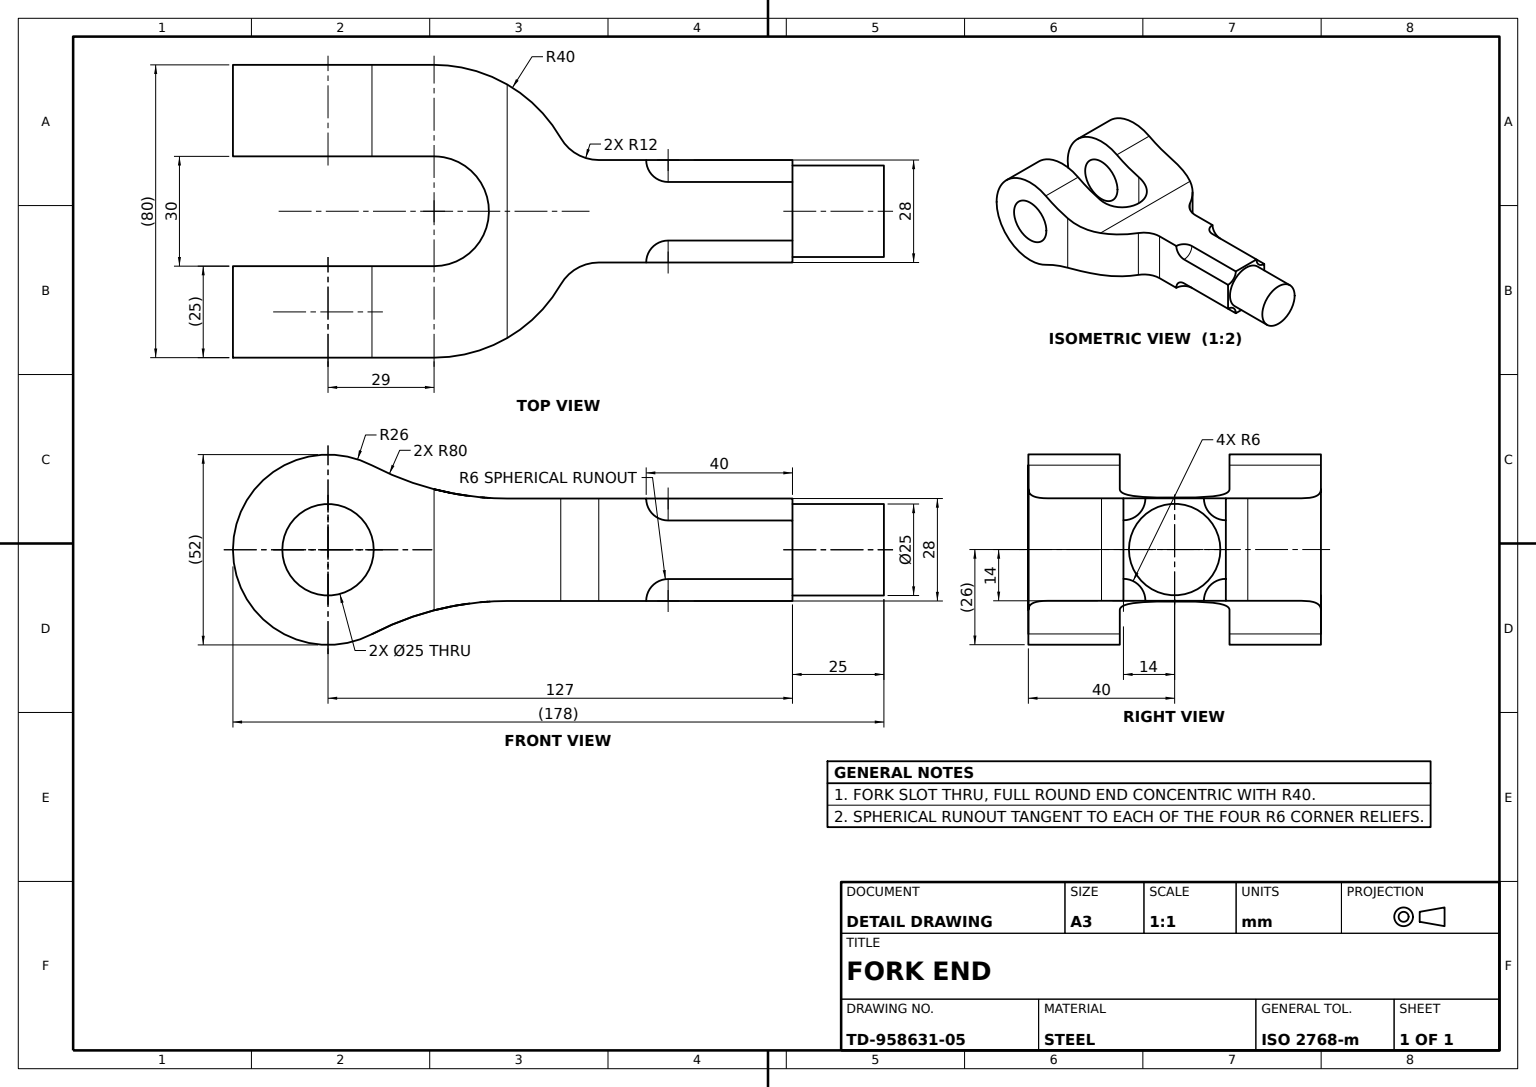
ISO-10303-21;
HEADER;
FILE_DESCRIPTION((''),'2;1');
FILE_NAME('','',(''),(''),'','','');
FILE_SCHEMA(('AUTOMOTIVE_DESIGN'));
ENDSEC;
DATA;
#1=APPLICATION_CONTEXT('');
#2=PRODUCT_CONTEXT('',#1,'mechanical');
#3=PRODUCT('','','',(#2));
#4=PRODUCT_DEFINITION_FORMATION('','',#3);
#5=PRODUCT_DEFINITION_CONTEXT('',#1,'design');
#6=PRODUCT_DEFINITION('','',#4,#5);
#7=PRODUCT_DEFINITION_SHAPE('','',#6);
#8=(LENGTH_UNIT()NAMED_UNIT(*)SI_UNIT(.MILLI.,.METRE.));
#9=(NAMED_UNIT(*)PLANE_ANGLE_UNIT()SI_UNIT($,.RADIAN.));
#10=(NAMED_UNIT(*)SI_UNIT($,.STERADIAN.)SOLID_ANGLE_UNIT());
#11=UNCERTAINTY_MEASURE_WITH_UNIT(LENGTH_MEASURE(1.E-05),#8,'distance_accuracy_value','');
#12=(GEOMETRIC_REPRESENTATION_CONTEXT(3)GLOBAL_UNCERTAINTY_ASSIGNED_CONTEXT((#11))GLOBAL_UNIT_ASSIGNED_CONTEXT((#8,#9,#10))REPRESENTATION_CONTEXT('',''));
#13=CARTESIAN_POINT('',(0.,37.24122,-16.5));
#14=VERTEX_POINT('',#13);
#15=CARTESIAN_POINT('',(0.,37.24122,-41.5));
#16=VERTEX_POINT('',#15);
#17=CARTESIAN_POINT('',(0.,37.24122,-29.));
#18=DIRECTION('',(-1.,0.,0.));
#19=DIRECTION('',(0.,0.,1.));
#20=AXIS2_PLACEMENT_3D('',#17,#18,#19);
#21=CIRCLE('',#20,12.5);
#22=EDGE_CURVE('',#14,#16,#21,.T.);
#23=ORIENTED_EDGE('',*,*,#22,.T.);
#24=CARTESIAN_POINT('',(25.,37.24122,-41.5));
#25=VERTEX_POINT('',#24);
#26=CARTESIAN_POINT('',(80.,37.24122,-41.5));
#27=VECTOR('',#18,1000.);
#28=LINE('',#26,#27);
#29=EDGE_CURVE('',#25,#16,#28,.T.);
#30=ORIENTED_EDGE('',*,*,#29,.F.);
#31=CARTESIAN_POINT('',(25.,37.24122,-16.5));
#32=VERTEX_POINT('',#31);
#33=CARTESIAN_POINT('',(25.,37.24122,-29.));
#34=AXIS2_PLACEMENT_3D('',#33,#18,#19);
#35=CIRCLE('',#34,12.5);
#36=EDGE_CURVE('',#32,#25,#35,.T.);
#37=ORIENTED_EDGE('',*,*,#36,.F.);
#38=CARTESIAN_POINT('',(80.,37.24122,-16.5));
#39=LINE('',#38,#27);
#40=EDGE_CURVE('',#32,#14,#39,.T.);
#41=ORIENTED_EDGE('',*,*,#40,.T.);
#42=EDGE_LOOP('',(#23,#30,#37,#41));
#43=FACE_OUTER_BOUND('',#42,.T.);
#44=CARTESIAN_POINT('',(80.,37.24122,-29.));
#45=AXIS2_PLACEMENT_3D('',#44,#18,#19);
#46=CYLINDRICAL_SURFACE('',#45,12.5);
#47=ADVANCED_FACE('',(#43),#46,.F.);
#48=CARTESIAN_POINT('',(54.,23.24122,-116.));
#49=VERTEX_POINT('',#48);
#50=CARTESIAN_POINT('',(54.,29.24122,-122.));
#51=VERTEX_POINT('',#50);
#52=CARTESIAN_POINT('',(54.,23.24122,-122.));
#53=AXIS2_PLACEMENT_3D('',#52,#18,#19);
#54=CIRCLE('',#53,6.);
#55=EDGE_CURVE('',#49,#51,#54,.T.);
#56=ORIENTED_EDGE('',*,*,#55,.F.);
#57=CARTESIAN_POINT('',(48.,23.24122,-122.));
#58=VERTEX_POINT('',#57);
#59=DIRECTION('',(0.,1.,0.));
#60=DIRECTION('',(0.,0.,-1.));
#61=AXIS2_PLACEMENT_3D('',#52,#59,#60);
#62=CIRCLE('',#61,6.);
#63=EDGE_CURVE('',#58,#49,#62,.T.);
#64=ORIENTED_EDGE('',*,*,#63,.F.);
#65=AXIS2_PLACEMENT_3D('',#52,#19,#18);
#66=CIRCLE('',#65,6.);
#67=EDGE_CURVE('',#51,#58,#66,.T.);
#68=ORIENTED_EDGE('',*,*,#67,.F.);
#69=EDGE_LOOP('',(#56,#64,#68));
#70=FACE_OUTER_BOUND('',#69,.T.);
#71=AXIS2_PLACEMENT_3D('',#52,#59,#18);
#72=SPHERICAL_SURFACE('',#71,6.);
#73=ADVANCED_FACE('',(#70),#72,.F.);
#74=CARTESIAN_POINT('',(54.,45.24122,-156.));
#75=VERTEX_POINT('',#74);
#76=CARTESIAN_POINT('',(48.,51.24122,-156.));
#77=VERTEX_POINT('',#76);
#78=CARTESIAN_POINT('',(54.,51.24122,-156.));
#79=AXIS2_PLACEMENT_3D('',#78,#60,#18);
#80=CIRCLE('',#79,6.);
#81=EDGE_CURVE('',#75,#77,#80,.T.);
#82=ORIENTED_EDGE('',*,*,#81,.F.);
#83=CARTESIAN_POINT('',(54.,29.24122,-156.));
#84=VERTEX_POINT('',#83);
#85=CARTESIAN_POINT('',(54.,0.,-156.));
#86=VECTOR('',#59,1000.);
#87=LINE('',#85,#86);
#88=EDGE_CURVE('',#84,#75,#87,.T.);
#89=ORIENTED_EDGE('',*,*,#88,.F.);
#90=CARTESIAN_POINT('',(48.,23.24122,-156.));
#91=VERTEX_POINT('',#90);
#92=CARTESIAN_POINT('',(54.,23.24122,-156.));
#93=AXIS2_PLACEMENT_3D('',#92,#60,#18);
#94=CIRCLE('',#93,6.);
#95=EDGE_CURVE('',#91,#84,#94,.T.);
#96=ORIENTED_EDGE('',*,*,#95,.F.);
#97=CARTESIAN_POINT('',(32.,23.24122,-156.));
#98=VERTEX_POINT('',#97);
#99=CARTESIAN_POINT('',(80.,23.24122,-156.));
#100=LINE('',#99,#27);
#101=EDGE_CURVE('',#91,#98,#100,.T.);
#102=ORIENTED_EDGE('',*,*,#101,.T.);
#103=CARTESIAN_POINT('',(26.,29.24122,-156.));
#104=VERTEX_POINT('',#103);
#105=CARTESIAN_POINT('',(26.,23.24122,-156.));
#106=AXIS2_PLACEMENT_3D('',#105,#60,#18);
#107=CIRCLE('',#106,6.);
#108=EDGE_CURVE('',#104,#98,#107,.T.);
#109=ORIENTED_EDGE('',*,*,#108,.F.);
#110=CARTESIAN_POINT('',(26.,45.24122,-156.));
#111=VERTEX_POINT('',#110);
#112=CARTESIAN_POINT('',(26.,0.,-156.));
#113=LINE('',#112,#86);
#114=EDGE_CURVE('',#104,#111,#113,.T.);
#115=ORIENTED_EDGE('',*,*,#114,.T.);
#116=CARTESIAN_POINT('',(32.,51.24122,-156.));
#117=VERTEX_POINT('',#116);
#118=CARTESIAN_POINT('',(26.,51.24122,-156.));
#119=AXIS2_PLACEMENT_3D('',#118,#60,#18);
#120=CIRCLE('',#119,6.);
#121=EDGE_CURVE('',#117,#111,#120,.T.);
#122=ORIENTED_EDGE('',*,*,#121,.F.);
#123=CARTESIAN_POINT('',(80.,51.24122,-156.));
#124=LINE('',#123,#27);
#125=EDGE_CURVE('',#77,#117,#124,.T.);
#126=ORIENTED_EDGE('',*,*,#125,.F.);
#127=EDGE_LOOP('',(#82,#89,#96,#102,#109,#115,#122,#126));
#128=FACE_OUTER_BOUND('',#127,.T.);
#129=CARTESIAN_POINT('',(52.5,37.24122,-156.));
#130=VERTEX_POINT('',#129);
#131=CARTESIAN_POINT('',(27.5,37.24122,-156.));
#132=VERTEX_POINT('',#131);
#133=CARTESIAN_POINT('',(40.,37.24122,-156.));
#134=AXIS2_PLACEMENT_3D('',#133,#60,#18);
#135=CIRCLE('',#134,12.5);
#136=EDGE_CURVE('',#130,#132,#135,.T.);
#137=ORIENTED_EDGE('',*,*,#136,.F.);
#138=EDGE_CURVE('',#132,#130,#135,.T.);
#139=ORIENTED_EDGE('',*,*,#138,.F.);
#140=EDGE_LOOP('',(#137,#139));
#141=FACE_BOUND('',#140,.T.);
#142=CARTESIAN_POINT('',(0.,66.,-156.));
#143=DIRECTION('',(1.,0.,0.));
#144=AXIS2_PLACEMENT_3D('',#142,#19,#143);
#145=PLANE('',#144);
#146=ADVANCED_FACE('',(#128,#141),#145,.F.);
#147=ORIENTED_EDGE('',*,*,#67,.T.);
#148=CARTESIAN_POINT('',(48.,23.24122,-116.));
#149=VECTOR('',#60,1000.);
#150=LINE('',#148,#149);
#151=EDGE_CURVE('',#58,#91,#150,.T.);
#152=ORIENTED_EDGE('',*,*,#151,.T.);
#153=ORIENTED_EDGE('',*,*,#95,.T.);
#154=CARTESIAN_POINT('',(54.,29.24122,-116.));
#155=LINE('',#154,#149);
#156=EDGE_CURVE('',#51,#84,#155,.T.);
#157=ORIENTED_EDGE('',*,*,#156,.F.);
#158=EDGE_LOOP('',(#147,#152,#153,#157));
#159=FACE_OUTER_BOUND('',#158,.T.);
#160=AXIS2_PLACEMENT_3D('',#48,#60,#18);
#161=CYLINDRICAL_SURFACE('',#160,6.);
#162=ADVANCED_FACE('',(#159),#161,.F.);
#163=CARTESIAN_POINT('',(54.,51.24122,-116.));
#164=VERTEX_POINT('',#163);
#165=CARTESIAN_POINT('',(48.,51.24122,-122.));
#166=VERTEX_POINT('',#165);
#167=CARTESIAN_POINT('',(54.,51.24122,-122.));
#168=DIRECTION('',(0.,-1.,0.));
#169=AXIS2_PLACEMENT_3D('',#167,#168,#19);
#170=CIRCLE('',#169,6.);
#171=EDGE_CURVE('',#164,#166,#170,.T.);
#172=ORIENTED_EDGE('',*,*,#171,.F.);
#173=CARTESIAN_POINT('',(54.,45.24122,-122.));
#174=VERTEX_POINT('',#173);
#175=AXIS2_PLACEMENT_3D('',#167,#18,#19);
#176=CIRCLE('',#175,6.);
#177=EDGE_CURVE('',#174,#164,#176,.T.);
#178=ORIENTED_EDGE('',*,*,#177,.F.);
#179=AXIS2_PLACEMENT_3D('',#167,#19,#18);
#180=CIRCLE('',#179,6.);
#181=EDGE_CURVE('',#166,#174,#180,.T.);
#182=ORIENTED_EDGE('',*,*,#181,.F.);
#183=EDGE_LOOP('',(#172,#178,#182));
#184=FACE_OUTER_BOUND('',#183,.T.);
#185=AXIS2_PLACEMENT_3D('',#167,#59,#18);
#186=SPHERICAL_SURFACE('',#185,6.);
#187=ADVANCED_FACE('',(#184),#186,.F.);
#188=VERTEX_POINT('',#38);
#189=CARTESIAN_POINT('',(55.,37.24122,-16.5));
#190=VERTEX_POINT('',#189);
#191=EDGE_CURVE('',#188,#190,#39,.T.);
#192=ORIENTED_EDGE('',*,*,#191,.F.);
#193=VERTEX_POINT('',#26);
#194=CIRCLE('',#45,12.5);
#195=EDGE_CURVE('',#193,#188,#194,.T.);
#196=ORIENTED_EDGE('',*,*,#195,.F.);
#197=CARTESIAN_POINT('',(55.,37.24122,-41.5));
#198=VERTEX_POINT('',#197);
#199=EDGE_CURVE('',#193,#198,#28,.T.);
#200=ORIENTED_EDGE('',*,*,#199,.T.);
#201=CARTESIAN_POINT('',(55.,37.24122,-29.));
#202=AXIS2_PLACEMENT_3D('',#201,#18,#19);
#203=CIRCLE('',#202,12.5);
#204=EDGE_CURVE('',#198,#190,#203,.T.);
#205=ORIENTED_EDGE('',*,*,#204,.T.);
#206=EDGE_LOOP('',(#192,#196,#200,#205));
#207=FACE_OUTER_BOUND('',#206,.T.);
#208=ADVANCED_FACE('',(#207),#46,.F.);
#209=CARTESIAN_POINT('',(80.,37.24122,-3.));
#210=VERTEX_POINT('',#209);
#211=CARTESIAN_POINT('',(80.,14.184616,-41.016365));
#212=VERTEX_POINT('',#211);
#213=AXIS2_PLACEMENT_3D('',#44,#143,#60);
#214=CIRCLE('',#213,26.);
#215=EDGE_CURVE('',#210,#212,#214,.T.);
#216=ORIENTED_EDGE('',*,*,#215,.T.);
#217=CARTESIAN_POINT('',(80.,20.703521,-58.));
#218=VERTEX_POINT('',#217);
#219=CARTESIAN_POINT('',(80.,-56.75878,-77.989795));
#220=AXIS2_PLACEMENT_3D('',#219,#143,#60);
#221=CIRCLE('',#220,80.);
#222=EDGE_CURVE('',#218,#212,#221,.T.);
#223=ORIENTED_EDGE('',*,*,#222,.F.);
#224=CARTESIAN_POINT('',(80.,53.778919,-58.));
#225=VERTEX_POINT('',#224);
#226=CARTESIAN_POINT('',(80.,0.,-58.));
#227=LINE('',#226,#86);
#228=EDGE_CURVE('',#218,#225,#227,.T.);
#229=ORIENTED_EDGE('',*,*,#228,.T.);
#230=CARTESIAN_POINT('',(80.,60.297824,-41.016365));
#231=VERTEX_POINT('',#230);
#232=CARTESIAN_POINT('',(80.,131.24122,-77.989795));
#233=AXIS2_PLACEMENT_3D('',#232,#18,#60);
#234=CIRCLE('',#233,80.);
#235=EDGE_CURVE('',#225,#231,#234,.T.);
#236=ORIENTED_EDGE('',*,*,#235,.T.);
#237=EDGE_CURVE('',#231,#210,#214,.T.);
#238=ORIENTED_EDGE('',*,*,#237,.T.);
#239=EDGE_LOOP('',(#216,#223,#229,#236,#238));
#240=FACE_OUTER_BOUND('',#239,.T.);
#241=EDGE_CURVE('',#188,#193,#194,.T.);
#242=ORIENTED_EDGE('',*,*,#241,.T.);
#243=ORIENTED_EDGE('',*,*,#195,.T.);
#244=EDGE_LOOP('',(#242,#243));
#245=FACE_BOUND('',#244,.T.);
#246=CARTESIAN_POINT('',(80.,66.,0.));
#247=AXIS2_PLACEMENT_3D('',#246,#18,#19);
#248=PLANE('',#247);
#249=ADVANCED_FACE('',(#240,#245),#248,.F.);
#250=CARTESIAN_POINT('',(25.,14.184616,-41.016365));
#251=VERTEX_POINT('',#250);
#252=CARTESIAN_POINT('',(0.,14.184616,-41.016365));
#253=VERTEX_POINT('',#252);
#254=LINE('',#211,#27);
#255=EDGE_CURVE('',#251,#253,#254,.T.);
#256=ORIENTED_EDGE('',*,*,#255,.T.);
#257=CARTESIAN_POINT('',(0.,20.703521,-58.));
#258=VERTEX_POINT('',#257);
#259=CARTESIAN_POINT('',(0.,-56.75878,-77.989795));
#260=AXIS2_PLACEMENT_3D('',#259,#143,#60);
#261=CIRCLE('',#260,80.);
#262=EDGE_CURVE('',#258,#253,#261,.T.);
#263=ORIENTED_EDGE('',*,*,#262,.F.);
#264=CARTESIAN_POINT('',(5.353094,23.24122,-77.989795));
#265=VERTEX_POINT('',#264);
#266=CARTESIAN_POINT('',(4.466039,23.24122,-76.452324));
#267=CARTESIAN_POINT('',(3.691516,23.196926,-74.874517));
#268=CARTESIAN_POINT('',(2.357938,23.005483,-71.642966));
#269=CARTESIAN_POINT('',(1.798915,22.858392,-69.989206));
#270=CARTESIAN_POINT('',(1.122963,22.548739,-67.45209));
#271=CARTESIAN_POINT('',(0.924277,22.430161,-66.593863));
#272=CARTESIAN_POINT('',(0.585664,22.163834,-64.875808));
#273=CARTESIAN_POINT('',(0.445574,22.016294,-64.016516));
#274=CARTESIAN_POINT('',(0.11037,21.529831,-61.438272));
#275=CARTESIAN_POINT('',(0.,21.147117,-59.718975));
#276=B_SPLINE_CURVE_WITH_KNOTS('',3,(#264,#266,#267,#268,#269,#270,#271,#272,#273,#274,#275,#257),.UNSPECIFIED.,.F.,.F.,(4,2,2,2,2,4),(0.,0.005250012,0.010500023,0.013125029,0.015750035,0.021000046),.UNSPECIFIED.);
#277=EDGE_CURVE('',#265,#258,#276,.T.);
#278=ORIENTED_EDGE('',*,*,#277,.F.);
#279=CARTESIAN_POINT('',(74.646906,23.24122,-77.989795));
#280=VERTEX_POINT('',#279);
#281=CARTESIAN_POINT('',(80.,23.24122,-77.989795));
#282=LINE('',#281,#27);
#283=EDGE_CURVE('',#280,#265,#282,.T.);
#284=ORIENTED_EDGE('',*,*,#283,.F.);
#285=CARTESIAN_POINT('',(80.,21.147039,-59.718673));
#286=CARTESIAN_POINT('',(79.88966,21.528128,-61.431544));
#287=CARTESIAN_POINT('',(79.447645,22.172901,-64.844255));
#288=CARTESIAN_POINT('',(79.116002,22.436561,-66.544103));
#289=CARTESIAN_POINT('',(78.444168,22.748317,-69.082049));
#290=CARTESIAN_POINT('',(78.190013,22.838512,-69.92902));
#291=CARTESIAN_POINT('',(77.626826,22.990167,-71.601491));
#292=CARTESIAN_POINT('',(77.318213,23.051717,-72.426575));
#293=CARTESIAN_POINT('',(76.311916,23.196937,-74.86846));
#294=CARTESIAN_POINT('',(75.534121,23.24122,-76.452048));
#295=B_SPLINE_CURVE_WITH_KNOTS('',3,(#217,#285,#286,#287,#288,#289,#290,#291,#292,#293,#294,#279),.UNSPECIFIED.,.F.,.F.,(4,2,2,2,2,4),(0.,0.005249947,0.010499894,0.013124868,0.015749841,0.020999788),.UNSPECIFIED.);
#296=EDGE_CURVE('',#218,#280,#295,.T.);
#297=ORIENTED_EDGE('',*,*,#296,.F.);
#298=ORIENTED_EDGE('',*,*,#222,.T.);
#299=CARTESIAN_POINT('',(55.,14.184616,-41.016365));
#300=VERTEX_POINT('',#299);
#301=EDGE_CURVE('',#212,#300,#254,.T.);
#302=ORIENTED_EDGE('',*,*,#301,.T.);
#303=CARTESIAN_POINT('',(55.,20.703521,-58.));
#304=VERTEX_POINT('',#303);
#305=CARTESIAN_POINT('',(55.,-56.75878,-77.989795));
#306=AXIS2_PLACEMENT_3D('',#305,#143,#19);
#307=CIRCLE('',#306,80.);
#308=EDGE_CURVE('',#304,#300,#307,.T.);
#309=ORIENTED_EDGE('',*,*,#308,.F.);
#310=CARTESIAN_POINT('',(25.,20.703521,-58.));
#311=VERTEX_POINT('',#310);
#312=CARTESIAN_POINT('',(55.,20.953008,-58.966784));
#313=CARTESIAN_POINT('',(54.907376,21.180447,-59.922887));
#314=CARTESIAN_POINT('',(54.631178,21.491094,-61.34073));
#315=CARTESIAN_POINT('',(54.516083,21.589548,-61.810602));
#316=CARTESIAN_POINT('',(54.238222,21.776614,-62.744512));
#317=CARTESIAN_POINT('',(54.074568,21.86547,-63.210117));
#318=CARTESIAN_POINT('',(53.521163,22.112574,-64.567591));
#319=CARTESIAN_POINT('',(53.067491,22.253426,-65.429712));
#320=CARTESIAN_POINT('',(52.259374,22.435564,-66.657236));
#321=CARTESIAN_POINT('',(51.96791,22.491511,-67.056236));
#322=CARTESIAN_POINT('',(51.343174,22.59409,-67.827444));
#323=CARTESIAN_POINT('',(51.013971,22.6401,-68.194805));
#324=CARTESIAN_POINT('',(49.977386,22.764799,-69.243585));
#325=CARTESIAN_POINT('',(49.221486,22.830267,-69.872204));
#326=CARTESIAN_POINT('',(47.988025,22.909416,-70.705814));
#327=CARTESIAN_POINT('',(47.560018,22.932547,-70.96498));
#328=CARTESIAN_POINT('',(46.689628,22.972565,-71.434785));
#329=CARTESIAN_POINT('',(46.24493,22.989614,-71.647092));
#330=CARTESIAN_POINT('',(45.336825,23.01893,-72.027137));
#331=CARTESIAN_POINT('',(44.873419,23.031195,-72.194875));
#332=CARTESIAN_POINT('',(43.927642,23.051743,-72.485106));
#333=CARTESIAN_POINT('',(43.44253,23.060057,-72.608086));
#334=CARTESIAN_POINT('',(41.980233,23.079507,-72.901927));
#335=CARTESIAN_POINT('',(40.999496,23.085401,-72.999137));
#336=CARTESIAN_POINT('',(39.519797,23.085482,-73.000423));
#337=CARTESIAN_POINT('',(39.025121,23.084004,-72.976588));
#338=CARTESIAN_POINT('',(38.032789,23.077804,-72.878799));
#339=CARTESIAN_POINT('',(37.540282,23.073102,-72.805192));
#340=CARTESIAN_POINT('',(36.087436,23.053861,-72.514391));
#341=CARTESIAN_POINT('',(35.145523,23.034327,-72.227315));
#342=CARTESIAN_POINT('',(33.773131,22.990281,-71.655465));
#343=CARTESIAN_POINT('',(33.320594,22.972986,-71.439905));
#344=CARTESIAN_POINT('',(32.448192,22.932972,-70.9698));
#345=CARTESIAN_POINT('',(32.026329,22.910213,-70.714653));
#346=CARTESIAN_POINT('',(31.21069,22.858118,-70.165108));
#347=CARTESIAN_POINT('',(30.816915,22.828783,-69.870709));
#348=CARTESIAN_POINT('',(30.057683,22.762186,-69.242469));
#349=CARTESIAN_POINT('',(29.691283,22.724813,-68.907672));
#350=CARTESIAN_POINT('',(28.642243,22.598993,-67.848312));
#351=CARTESIAN_POINT('',(28.024683,22.498897,-67.085616));
#352=CARTESIAN_POINT('',(27.215853,22.31762,-65.861599));
#353=CARTESIAN_POINT('',(26.965968,22.251986,-65.440166));
#354=CARTESIAN_POINT('',(26.506443,22.108866,-64.570081));
#355=CARTESIAN_POINT('',(26.297409,22.031392,-64.121857));
#356=CARTESIAN_POINT('',(25.744032,21.784812,-62.766537));
#357=CARTESIAN_POINT('',(25.467399,21.600054,-61.839308));
#358=CARTESIAN_POINT('',(25.187727,21.288335,-60.414695));
#359=CARTESIAN_POINT('',(25.117077,21.178212,-59.93234));
#360=CARTESIAN_POINT('',(25.02332,20.948144,-58.966643));
#361=CARTESIAN_POINT('',(25.,20.828284,-58.483468));
#362=B_SPLINE_CURVE_WITH_KNOTS('',3,(#303,#312,#313,#314,#315,#316,#317,#318,#319,#320,#321,#322,#323,#324,#325,#326,#327,#328,#329,#330,#331,#332,#333,#334,#335,#336,#337,#338,#339,#340,#341,#342,#343,#344,#345,#346,#347,#348,#349,#350,#351,#352,#353,#354,#355,#356,#357,#358,#359,#360,#361,#310),.UNSPECIFIED.,.F.,.F.,(4,2,2,2,2,2,2,2,2,2,2,2,2,2,2,2,2,2,2,2,2,2,2,2,2,4),(0.,0.002954089,0.004431134,0.005908178,0.008862268,0.010339312,0.011816357,0.014770446,0.016247491,0.017724535,0.01920158,0.020678625,0.023632714,0.025109758,0.026586803,0.029540892,0.031017937,0.032494982,0.033972026,0.035449071,0.03840316,0.039880205,0.041357249,0.044311338,0.045788383,0.047265428),.UNSPECIFIED.);
#363=EDGE_CURVE('',#304,#311,#362,.T.);
#364=ORIENTED_EDGE('',*,*,#363,.T.);
#365=CARTESIAN_POINT('',(25.,-56.75878,-77.989795));
#366=AXIS2_PLACEMENT_3D('',#365,#143,#19);
#367=CIRCLE('',#366,80.);
#368=EDGE_CURVE('',#311,#251,#367,.T.);
#369=ORIENTED_EDGE('',*,*,#368,.T.);
#370=EDGE_LOOP('',(#256,#263,#278,#284,#297,#298,#302,#309,#364,#369));
#371=FACE_OUTER_BOUND('',#370,.T.);
#372=AXIS2_PLACEMENT_3D('',#219,#18,#19);
#373=CYLINDRICAL_SURFACE('',#372,80.);
#374=ADVANCED_FACE('',(#371),#373,.F.);
#375=ORIENTED_EDGE('',*,*,#121,.T.);
#376=CARTESIAN_POINT('',(26.,45.24122,-122.));
#377=VERTEX_POINT('',#376);
#378=CARTESIAN_POINT('',(26.,45.24122,-116.));
#379=VECTOR('',#19,1000.);
#380=LINE('',#378,#379);
#381=EDGE_CURVE('',#111,#377,#380,.T.);
#382=ORIENTED_EDGE('',*,*,#381,.T.);
#383=CARTESIAN_POINT('',(32.,51.24122,-122.));
#384=VERTEX_POINT('',#383);
#385=CARTESIAN_POINT('',(26.,51.24122,-122.));
#386=AXIS2_PLACEMENT_3D('',#385,#19,#18);
#387=CIRCLE('',#386,6.);
#388=EDGE_CURVE('',#377,#384,#387,.T.);
#389=ORIENTED_EDGE('',*,*,#388,.T.);
#390=CARTESIAN_POINT('',(32.,51.24122,-116.));
#391=LINE('',#390,#149);
#392=EDGE_CURVE('',#384,#117,#391,.T.);
#393=ORIENTED_EDGE('',*,*,#392,.T.);
#394=EDGE_LOOP('',(#375,#382,#389,#393));
#395=FACE_OUTER_BOUND('',#394,.T.);
#396=CARTESIAN_POINT('',(26.,51.24122,-116.));
#397=AXIS2_PLACEMENT_3D('',#396,#60,#18);
#398=CYLINDRICAL_SURFACE('',#397,6.);
#399=ADVANCED_FACE('',(#395),#398,.F.);
#400=VERTEX_POINT('',#396);
#401=AXIS2_PLACEMENT_3D('',#385,#168,#19);
#402=CIRCLE('',#401,6.);
#403=EDGE_CURVE('',#384,#400,#402,.T.);
#404=ORIENTED_EDGE('',*,*,#403,.F.);
#405=ORIENTED_EDGE('',*,*,#388,.F.);
#406=AXIS2_PLACEMENT_3D('',#385,#143,#19);
#407=CIRCLE('',#406,6.);
#408=EDGE_CURVE('',#400,#377,#407,.T.);
#409=ORIENTED_EDGE('',*,*,#408,.F.);
#410=EDGE_LOOP('',(#404,#405,#409));
#411=FACE_OUTER_BOUND('',#410,.T.);
#412=AXIS2_PLACEMENT_3D('',#385,#59,#18);
#413=SPHERICAL_SURFACE('',#412,6.);
#414=ADVANCED_FACE('',(#411),#413,.F.);
#415=CARTESIAN_POINT('',(55.,60.297824,-41.016365));
#416=VERTEX_POINT('',#415);
#417=LINE('',#230,#27);
#418=EDGE_CURVE('',#231,#416,#417,.T.);
#419=ORIENTED_EDGE('',*,*,#418,.T.);
#420=CARTESIAN_POINT('',(55.,37.24122,-3.));
#421=VERTEX_POINT('',#420);
#422=AXIS2_PLACEMENT_3D('',#201,#143,#19);
#423=CIRCLE('',#422,26.);
#424=EDGE_CURVE('',#416,#421,#423,.T.);
#425=ORIENTED_EDGE('',*,*,#424,.T.);
#426=LINE('',#209,#27);
#427=EDGE_CURVE('',#210,#421,#426,.T.);
#428=ORIENTED_EDGE('',*,*,#427,.F.);
#429=ORIENTED_EDGE('',*,*,#237,.F.);
#430=EDGE_LOOP('',(#419,#425,#428,#429));
#431=FACE_OUTER_BOUND('',#430,.T.);
#432=CYLINDRICAL_SURFACE('',#45,26.);
#433=ADVANCED_FACE('',(#431),#432,.T.);
#434=ORIENTED_EDGE('',*,*,#255,.F.);
#435=CARTESIAN_POINT('',(25.,37.24122,-3.));
#436=VERTEX_POINT('',#435);
#437=AXIS2_PLACEMENT_3D('',#33,#143,#19);
#438=CIRCLE('',#437,26.);
#439=EDGE_CURVE('',#436,#251,#438,.T.);
#440=ORIENTED_EDGE('',*,*,#439,.F.);
#441=CARTESIAN_POINT('',(0.,37.24122,-3.));
#442=VERTEX_POINT('',#441);
#443=EDGE_CURVE('',#436,#442,#426,.T.);
#444=ORIENTED_EDGE('',*,*,#443,.T.);
#445=AXIS2_PLACEMENT_3D('',#17,#143,#60);
#446=CIRCLE('',#445,26.);
#447=EDGE_CURVE('',#442,#253,#446,.T.);
#448=ORIENTED_EDGE('',*,*,#447,.T.);
#449=EDGE_LOOP('',(#434,#440,#444,#448));
#450=FACE_OUTER_BOUND('',#449,.T.);
#451=ADVANCED_FACE('',(#450),#432,.T.);
#452=ORIENTED_EDGE('',*,*,#301,.F.);
#453=ORIENTED_EDGE('',*,*,#215,.F.);
#454=ORIENTED_EDGE('',*,*,#427,.T.);
#455=EDGE_CURVE('',#421,#300,#423,.T.);
#456=ORIENTED_EDGE('',*,*,#455,.T.);
#457=EDGE_LOOP('',(#452,#453,#454,#456));
#458=FACE_OUTER_BOUND('',#457,.T.);
#459=ADVANCED_FACE('',(#458),#432,.T.);
#460=ORIENTED_EDGE('',*,*,#114,.F.);
#461=CARTESIAN_POINT('',(26.,29.24122,-122.));
#462=VERTEX_POINT('',#461);
#463=CARTESIAN_POINT('',(26.,29.24122,-116.));
#464=LINE('',#463,#149);
#465=EDGE_CURVE('',#462,#104,#464,.T.);
#466=ORIENTED_EDGE('',*,*,#465,.F.);
#467=CARTESIAN_POINT('',(26.,23.24122,-116.));
#468=VERTEX_POINT('',#467);
#469=CARTESIAN_POINT('',(26.,23.24122,-122.));
#470=AXIS2_PLACEMENT_3D('',#469,#143,#19);
#471=CIRCLE('',#470,6.);
#472=EDGE_CURVE('',#462,#468,#471,.T.);
#473=ORIENTED_EDGE('',*,*,#472,.T.);
#474=CARTESIAN_POINT('',(26.,23.24122,-103.033321));
#475=VERTEX_POINT('',#474);
#476=CARTESIAN_POINT('',(26.,23.24122,0.));
#477=LINE('',#476,#379);
#478=EDGE_CURVE('',#468,#475,#477,.T.);
#479=ORIENTED_EDGE('',*,*,#478,.T.);
#480=CARTESIAN_POINT('',(26.,51.24122,-103.033321));
#481=VERTEX_POINT('',#480);
#482=CARTESIAN_POINT('',(26.,0.,-103.033321));
#483=LINE('',#482,#86);
#484=EDGE_CURVE('',#475,#481,#483,.T.);
#485=ORIENTED_EDGE('',*,*,#484,.T.);
#486=CARTESIAN_POINT('',(26.,51.24122,0.));
#487=LINE('',#486,#149);
#488=EDGE_CURVE('',#481,#400,#487,.T.);
#489=ORIENTED_EDGE('',*,*,#488,.T.);
#490=ORIENTED_EDGE('',*,*,#408,.T.);
#491=ORIENTED_EDGE('',*,*,#381,.F.);
#492=EDGE_LOOP('',(#460,#466,#473,#479,#485,#489,#490,#491));
#493=FACE_OUTER_BOUND('',#492,.T.);
#494=CARTESIAN_POINT('',(26.,0.,0.));
#495=AXIS2_PLACEMENT_3D('',#494,#18,#19);
#496=PLANE('',#495);
#497=ADVANCED_FACE('',(#493),#496,.T.);
#498=ORIENTED_EDGE('',*,*,#277,.T.);
#499=CARTESIAN_POINT('',(0.,53.778919,-58.));
#500=VERTEX_POINT('',#499);
#501=CARTESIAN_POINT('',(0.,0.,-58.));
#502=LINE('',#501,#86);
#503=EDGE_CURVE('',#258,#500,#502,.T.);
#504=ORIENTED_EDGE('',*,*,#503,.T.);
#505=CARTESIAN_POINT('',(5.353094,51.24122,-77.989795));
#506=VERTEX_POINT('',#505);
#507=CARTESIAN_POINT('',(4.466039,51.24122,-76.452324));
#508=CARTESIAN_POINT('',(3.691516,51.285514,-74.874517));
#509=CARTESIAN_POINT('',(2.357938,51.476957,-71.642966));
#510=CARTESIAN_POINT('',(1.798915,51.624048,-69.989206));
#511=CARTESIAN_POINT('',(1.122963,51.9337,-67.45209));
#512=CARTESIAN_POINT('',(0.924277,52.052279,-66.593863));
#513=CARTESIAN_POINT('',(0.585664,52.318606,-64.875808));
#514=CARTESIAN_POINT('',(0.445574,52.466145,-64.016516));
#515=CARTESIAN_POINT('',(0.11037,52.952609,-61.438272));
#516=CARTESIAN_POINT('',(0.,53.335323,-59.718975));
#517=B_SPLINE_CURVE_WITH_KNOTS('',3,(#505,#507,#508,#509,#510,#511,#512,#513,#514,#515,#516,#499),.UNSPECIFIED.,.F.,.F.,(4,2,2,2,2,4),(0.,0.005250012,0.010500023,0.013125029,0.015750035,0.021000046),.UNSPECIFIED.);
#518=EDGE_CURVE('',#506,#500,#517,.T.);
#519=ORIENTED_EDGE('',*,*,#518,.F.);
#520=CARTESIAN_POINT('',(20.,51.24122,-92.641016));
#521=VERTEX_POINT('',#520);
#522=CARTESIAN_POINT('',(40.,51.24122,-58.));
#523=AXIS2_PLACEMENT_3D('',#522,#168,#19);
#524=CIRCLE('',#523,40.);
#525=EDGE_CURVE('',#506,#521,#524,.T.);
#526=ORIENTED_EDGE('',*,*,#525,.T.);
#527=CARTESIAN_POINT('',(20.,23.24122,-92.641016));
#528=VERTEX_POINT('',#527);
#529=CARTESIAN_POINT('',(20.,0.,-92.641016));
#530=LINE('',#529,#86);
#531=EDGE_CURVE('',#528,#521,#530,.T.);
#532=ORIENTED_EDGE('',*,*,#531,.F.);
#533=CARTESIAN_POINT('',(40.,23.24122,-58.));
#534=AXIS2_PLACEMENT_3D('',#533,#59,#60);
#535=CIRCLE('',#534,40.);
#536=EDGE_CURVE('',#528,#265,#535,.T.);
#537=ORIENTED_EDGE('',*,*,#536,.T.);
#538=EDGE_LOOP('',(#498,#504,#519,#526,#532,#537));
#539=FACE_OUTER_BOUND('',#538,.T.);
#540=CARTESIAN_POINT('',(40.,0.,-58.));
#541=AXIS2_PLACEMENT_3D('',#540,#59,#19);
#542=CYLINDRICAL_SURFACE('',#541,40.);
#543=ADVANCED_FACE('',(#539),#542,.T.);
#544=ORIENTED_EDGE('',*,*,#424,.F.);
#545=CARTESIAN_POINT('',(55.,53.778919,-58.));
#546=VERTEX_POINT('',#545);
#547=CARTESIAN_POINT('',(55.,131.24122,-77.989795));
#548=AXIS2_PLACEMENT_3D('',#547,#18,#19);
#549=CIRCLE('',#548,80.);
#550=EDGE_CURVE('',#546,#416,#549,.T.);
#551=ORIENTED_EDGE('',*,*,#550,.F.);
#552=CARTESIAN_POINT('',(55.,0.,-58.));
#553=LINE('',#552,#86);
#554=EDGE_CURVE('',#304,#546,#553,.T.);
#555=ORIENTED_EDGE('',*,*,#554,.F.);
#556=ORIENTED_EDGE('',*,*,#308,.T.);
#557=ORIENTED_EDGE('',*,*,#455,.F.);
#558=EDGE_LOOP('',(#544,#551,#555,#556,#557));
#559=FACE_OUTER_BOUND('',#558,.T.);
#560=EDGE_CURVE('',#190,#198,#203,.T.);
#561=ORIENTED_EDGE('',*,*,#560,.F.);
#562=ORIENTED_EDGE('',*,*,#204,.F.);
#563=EDGE_LOOP('',(#561,#562));
#564=FACE_BOUND('',#563,.T.);
#565=CARTESIAN_POINT('',(55.,0.,0.));
#566=AXIS2_PLACEMENT_3D('',#565,#18,#19);
#567=PLANE('',#566);
#568=ADVANCED_FACE('',(#559,#564),#567,.T.);
#569=ORIENTED_EDGE('',*,*,#156,.T.);
#570=ORIENTED_EDGE('',*,*,#88,.T.);
#571=CARTESIAN_POINT('',(54.,45.24122,-116.));
#572=LINE('',#571,#379);
#573=EDGE_CURVE('',#75,#174,#572,.T.);
#574=ORIENTED_EDGE('',*,*,#573,.T.);
#575=ORIENTED_EDGE('',*,*,#177,.T.);
#576=CARTESIAN_POINT('',(54.,51.24122,-103.033321));
#577=VERTEX_POINT('',#576);
#578=CARTESIAN_POINT('',(54.,51.24122,0.));
#579=LINE('',#578,#149);
#580=EDGE_CURVE('',#577,#164,#579,.T.);
#581=ORIENTED_EDGE('',*,*,#580,.F.);
#582=CARTESIAN_POINT('',(54.,23.24122,-103.033321));
#583=VERTEX_POINT('',#582);
#584=CARTESIAN_POINT('',(54.,0.,-103.033321));
#585=LINE('',#584,#86);
#586=EDGE_CURVE('',#583,#577,#585,.T.);
#587=ORIENTED_EDGE('',*,*,#586,.F.);
#588=CARTESIAN_POINT('',(54.,23.24122,0.));
#589=LINE('',#588,#379);
#590=EDGE_CURVE('',#49,#583,#589,.T.);
#591=ORIENTED_EDGE('',*,*,#590,.F.);
#592=ORIENTED_EDGE('',*,*,#55,.T.);
#593=EDGE_LOOP('',(#569,#570,#574,#575,#581,#587,#591,#592));
#594=FACE_OUTER_BOUND('',#593,.T.);
#595=CARTESIAN_POINT('',(54.,0.,0.));
#596=AXIS2_PLACEMENT_3D('',#595,#18,#19);
#597=PLANE('',#596);
#598=ADVANCED_FACE('',(#594),#597,.F.);
#599=CARTESIAN_POINT('',(52.5,37.24122,-181.));
#600=VERTEX_POINT('',#599);
#601=CARTESIAN_POINT('',(27.5,37.24122,-181.));
#602=VERTEX_POINT('',#601);
#603=CARTESIAN_POINT('',(40.,37.24122,-181.));
#604=AXIS2_PLACEMENT_3D('',#603,#60,#18);
#605=CIRCLE('',#604,12.5);
#606=EDGE_CURVE('',#600,#602,#605,.T.);
#607=ORIENTED_EDGE('',*,*,#606,.F.);
#608=LINE('',#599,#379);
#609=EDGE_CURVE('',#600,#130,#608,.T.);
#610=ORIENTED_EDGE('',*,*,#609,.T.);
#611=ORIENTED_EDGE('',*,*,#136,.T.);
#612=LINE('',#601,#379);
#613=EDGE_CURVE('',#602,#132,#612,.T.);
#614=ORIENTED_EDGE('',*,*,#613,.F.);
#615=EDGE_LOOP('',(#607,#610,#611,#614));
#616=FACE_OUTER_BOUND('',#615,.T.);
#617=AXIS2_PLACEMENT_3D('',#603,#19,#143);
#618=CYLINDRICAL_SURFACE('',#617,12.5);
#619=ADVANCED_FACE('',(#616),#618,.T.);
#620=EDGE_CURVE('',#25,#32,#35,.T.);
#621=ORIENTED_EDGE('',*,*,#620,.F.);
#622=ORIENTED_EDGE('',*,*,#29,.T.);
#623=EDGE_CURVE('',#16,#14,#21,.T.);
#624=ORIENTED_EDGE('',*,*,#623,.T.);
#625=ORIENTED_EDGE('',*,*,#40,.F.);
#626=EDGE_LOOP('',(#621,#622,#624,#625));
#627=FACE_OUTER_BOUND('',#626,.T.);
#628=ADVANCED_FACE('',(#627),#46,.F.);
#629=ORIENTED_EDGE('',*,*,#439,.T.);
#630=ORIENTED_EDGE('',*,*,#368,.F.);
#631=CARTESIAN_POINT('',(25.,53.778919,-58.));
#632=VERTEX_POINT('',#631);
#633=CARTESIAN_POINT('',(25.,0.,-58.));
#634=LINE('',#633,#86);
#635=EDGE_CURVE('',#311,#632,#634,.T.);
#636=ORIENTED_EDGE('',*,*,#635,.T.);
#637=CARTESIAN_POINT('',(25.,60.297824,-41.016365));
#638=VERTEX_POINT('',#637);
#639=CARTESIAN_POINT('',(25.,131.24122,-77.989795));
#640=AXIS2_PLACEMENT_3D('',#639,#18,#19);
#641=CIRCLE('',#640,80.);
#642=EDGE_CURVE('',#632,#638,#641,.T.);
#643=ORIENTED_EDGE('',*,*,#642,.T.);
#644=EDGE_CURVE('',#638,#436,#438,.T.);
#645=ORIENTED_EDGE('',*,*,#644,.T.);
#646=EDGE_LOOP('',(#629,#630,#636,#643,#645));
#647=FACE_OUTER_BOUND('',#646,.T.);
#648=ORIENTED_EDGE('',*,*,#36,.T.);
#649=ORIENTED_EDGE('',*,*,#620,.T.);
#650=EDGE_LOOP('',(#648,#649));
#651=FACE_BOUND('',#650,.T.);
#652=CARTESIAN_POINT('',(25.,0.,0.));
#653=AXIS2_PLACEMENT_3D('',#652,#18,#19);
#654=PLANE('',#653);
#655=ADVANCED_FACE('',(#647,#651),#654,.F.);
#656=ORIENTED_EDGE('',*,*,#171,.T.);
#657=CARTESIAN_POINT('',(48.,51.24122,-116.));
#658=LINE('',#657,#379);
#659=EDGE_CURVE('',#77,#166,#658,.T.);
#660=ORIENTED_EDGE('',*,*,#659,.F.);
#661=ORIENTED_EDGE('',*,*,#125,.T.);
#662=ORIENTED_EDGE('',*,*,#392,.F.);
#663=ORIENTED_EDGE('',*,*,#403,.T.);
#664=ORIENTED_EDGE('',*,*,#488,.F.);
#665=CARTESIAN_POINT('',(14.,51.24122,-103.033321));
#666=AXIS2_PLACEMENT_3D('',#665,#59,#19);
#667=CIRCLE('',#666,12.);
#668=EDGE_CURVE('',#521,#481,#667,.T.);
#669=ORIENTED_EDGE('',*,*,#668,.F.);
#670=ORIENTED_EDGE('',*,*,#525,.F.);
#671=CARTESIAN_POINT('',(74.646906,51.24122,-77.989795));
#672=VERTEX_POINT('',#671);
#673=CARTESIAN_POINT('',(80.,51.24122,-77.989795));
#674=LINE('',#673,#27);
#675=EDGE_CURVE('',#672,#506,#674,.T.);
#676=ORIENTED_EDGE('',*,*,#675,.F.);
#677=CARTESIAN_POINT('',(60.,51.24122,-92.641016));
#678=VERTEX_POINT('',#677);
#679=EDGE_CURVE('',#678,#672,#524,.T.);
#680=ORIENTED_EDGE('',*,*,#679,.F.);
#681=CARTESIAN_POINT('',(66.,51.24122,-103.033321));
#682=AXIS2_PLACEMENT_3D('',#681,#168,#19);
#683=CIRCLE('',#682,12.);
#684=EDGE_CURVE('',#678,#577,#683,.T.);
#685=ORIENTED_EDGE('',*,*,#684,.T.);
#686=ORIENTED_EDGE('',*,*,#580,.T.);
#687=EDGE_LOOP('',(#656,#660,#661,#662,#663,#664,#669,#670,#676,#680,#685,#686));
#688=FACE_OUTER_BOUND('',#687,.T.);
#689=CARTESIAN_POINT('',(80.,51.24122,0.));
#690=AXIS2_PLACEMENT_3D('',#689,#59,#19);
#691=PLANE('',#690);
#692=ADVANCED_FACE('',(#688),#691,.T.);
#693=ORIENTED_EDGE('',*,*,#465,.T.);
#694=ORIENTED_EDGE('',*,*,#108,.T.);
#695=CARTESIAN_POINT('',(32.,23.24122,-122.));
#696=VERTEX_POINT('',#695);
#697=CARTESIAN_POINT('',(32.,23.24122,-116.));
#698=LINE('',#697,#379);
#699=EDGE_CURVE('',#98,#696,#698,.T.);
#700=ORIENTED_EDGE('',*,*,#699,.T.);
#701=AXIS2_PLACEMENT_3D('',#469,#19,#18);
#702=CIRCLE('',#701,6.);
#703=EDGE_CURVE('',#696,#462,#702,.T.);
#704=ORIENTED_EDGE('',*,*,#703,.T.);
#705=EDGE_LOOP('',(#693,#694,#700,#704));
#706=FACE_OUTER_BOUND('',#705,.T.);
#707=AXIS2_PLACEMENT_3D('',#467,#60,#18);
#708=CYLINDRICAL_SURFACE('',#707,6.);
#709=ADVANCED_FACE('',(#706),#708,.F.);
#710=CARTESIAN_POINT('',(60.,23.24122,-92.641016));
#711=VERTEX_POINT('',#710);
#712=CARTESIAN_POINT('',(60.,0.,-92.641016));
#713=LINE('',#712,#86);
#714=EDGE_CURVE('',#711,#678,#713,.T.);
#715=ORIENTED_EDGE('',*,*,#714,.F.);
#716=CARTESIAN_POINT('',(66.,23.24122,-103.033321));
#717=AXIS2_PLACEMENT_3D('',#716,#59,#60);
#718=CIRCLE('',#717,12.);
#719=EDGE_CURVE('',#583,#711,#718,.T.);
#720=ORIENTED_EDGE('',*,*,#719,.F.);
#721=ORIENTED_EDGE('',*,*,#586,.T.);
#722=ORIENTED_EDGE('',*,*,#684,.F.);
#723=EDGE_LOOP('',(#715,#720,#721,#722));
#724=FACE_OUTER_BOUND('',#723,.T.);
#725=CARTESIAN_POINT('',(66.,0.,-103.033321));
#726=AXIS2_PLACEMENT_3D('',#725,#59,#19);
#727=CYLINDRICAL_SURFACE('',#726,12.);
#728=ADVANCED_FACE('',(#724),#727,.F.);
#729=ORIENTED_EDGE('',*,*,#659,.T.);
#730=ORIENTED_EDGE('',*,*,#181,.T.);
#731=ORIENTED_EDGE('',*,*,#573,.F.);
#732=ORIENTED_EDGE('',*,*,#81,.T.);
#733=EDGE_LOOP('',(#729,#730,#731,#732));
#734=FACE_OUTER_BOUND('',#733,.T.);
#735=AXIS2_PLACEMENT_3D('',#163,#60,#18);
#736=CYLINDRICAL_SURFACE('',#735,6.);
#737=ADVANCED_FACE('',(#734),#736,.F.);
#738=CARTESIAN_POINT('',(0.,60.297824,-41.016365));
#739=VERTEX_POINT('',#738);
#740=EDGE_CURVE('',#739,#442,#446,.T.);
#741=ORIENTED_EDGE('',*,*,#740,.T.);
#742=ORIENTED_EDGE('',*,*,#443,.F.);
#743=ORIENTED_EDGE('',*,*,#644,.F.);
#744=EDGE_CURVE('',#638,#739,#417,.T.);
#745=ORIENTED_EDGE('',*,*,#744,.T.);
#746=EDGE_LOOP('',(#741,#742,#743,#745));
#747=FACE_OUTER_BOUND('',#746,.T.);
#748=ADVANCED_FACE('',(#747),#432,.T.);
#749=CARTESIAN_POINT('',(0.,131.24122,-77.989795));
#750=AXIS2_PLACEMENT_3D('',#749,#18,#60);
#751=CIRCLE('',#750,80.);
#752=EDGE_CURVE('',#500,#739,#751,.T.);
#753=ORIENTED_EDGE('',*,*,#752,.F.);
#754=ORIENTED_EDGE('',*,*,#503,.F.);
#755=ORIENTED_EDGE('',*,*,#262,.T.);
#756=ORIENTED_EDGE('',*,*,#447,.F.);
#757=ORIENTED_EDGE('',*,*,#740,.F.);
#758=EDGE_LOOP('',(#753,#754,#755,#756,#757));
#759=FACE_OUTER_BOUND('',#758,.T.);
#760=ORIENTED_EDGE('',*,*,#623,.F.);
#761=ORIENTED_EDGE('',*,*,#22,.F.);
#762=EDGE_LOOP('',(#760,#761));
#763=FACE_BOUND('',#762,.T.);
#764=CARTESIAN_POINT('',(0.,66.,0.));
#765=AXIS2_PLACEMENT_3D('',#764,#143,#60);
#766=PLANE('',#765);
#767=ADVANCED_FACE('',(#759,#763),#766,.F.);
#768=ORIENTED_EDGE('',*,*,#484,.F.);
#769=CARTESIAN_POINT('',(14.,23.24122,-103.033321));
#770=AXIS2_PLACEMENT_3D('',#769,#168,#60);
#771=CIRCLE('',#770,12.);
#772=EDGE_CURVE('',#475,#528,#771,.T.);
#773=ORIENTED_EDGE('',*,*,#772,.T.);
#774=ORIENTED_EDGE('',*,*,#531,.T.);
#775=ORIENTED_EDGE('',*,*,#668,.T.);
#776=EDGE_LOOP('',(#768,#773,#774,#775));
#777=FACE_OUTER_BOUND('',#776,.T.);
#778=CARTESIAN_POINT('',(14.,0.,-103.033321));
#779=AXIS2_PLACEMENT_3D('',#778,#59,#19);
#780=CYLINDRICAL_SURFACE('',#779,12.);
#781=ADVANCED_FACE('',(#777),#780,.F.);
#782=CARTESIAN_POINT('',(80.,53.335401,-59.718673));
#783=CARTESIAN_POINT('',(79.88966,52.954312,-61.431544));
#784=CARTESIAN_POINT('',(79.447645,52.309538,-64.844255));
#785=CARTESIAN_POINT('',(79.116002,52.045879,-66.544103));
#786=CARTESIAN_POINT('',(78.444168,51.734122,-69.082049));
#787=CARTESIAN_POINT('',(78.190013,51.643927,-69.92902));
#788=CARTESIAN_POINT('',(77.626826,51.492272,-71.601491));
#789=CARTESIAN_POINT('',(77.318213,51.430723,-72.426575));
#790=CARTESIAN_POINT('',(76.311916,51.285502,-74.86846));
#791=CARTESIAN_POINT('',(75.534121,51.24122,-76.452048));
#792=B_SPLINE_CURVE_WITH_KNOTS('',3,(#224,#782,#783,#784,#785,#786,#787,#788,#789,#790,#791,#671),.UNSPECIFIED.,.F.,.F.,(4,2,2,2,2,4),(0.,0.005249947,0.010499894,0.013124868,0.015749841,0.020999788),.UNSPECIFIED.);
#793=EDGE_CURVE('',#225,#672,#792,.T.);
#794=ORIENTED_EDGE('',*,*,#793,.T.);
#795=ORIENTED_EDGE('',*,*,#675,.T.);
#796=ORIENTED_EDGE('',*,*,#518,.T.);
#797=ORIENTED_EDGE('',*,*,#752,.T.);
#798=ORIENTED_EDGE('',*,*,#744,.F.);
#799=ORIENTED_EDGE('',*,*,#642,.F.);
#800=CARTESIAN_POINT('',(55.,53.529432,-58.966784));
#801=CARTESIAN_POINT('',(54.907376,53.301992,-59.922887));
#802=CARTESIAN_POINT('',(54.631178,52.991346,-61.34073));
#803=CARTESIAN_POINT('',(54.516083,52.892892,-61.810602));
#804=CARTESIAN_POINT('',(54.238222,52.705826,-62.744512));
#805=CARTESIAN_POINT('',(54.074568,52.61697,-63.210117));
#806=CARTESIAN_POINT('',(53.521163,52.369865,-64.567591));
#807=CARTESIAN_POINT('',(53.067491,52.229013,-65.429712));
#808=CARTESIAN_POINT('',(52.259374,52.046875,-66.657236));
#809=CARTESIAN_POINT('',(51.96791,51.990929,-67.056236));
#810=CARTESIAN_POINT('',(51.343174,51.88835,-67.827444));
#811=CARTESIAN_POINT('',(51.013971,51.84234,-68.194805));
#812=CARTESIAN_POINT('',(49.977386,51.717641,-69.243585));
#813=CARTESIAN_POINT('',(49.221486,51.652173,-69.872204));
#814=CARTESIAN_POINT('',(47.988025,51.573023,-70.705814));
#815=CARTESIAN_POINT('',(47.560018,51.549893,-70.96498));
#816=CARTESIAN_POINT('',(46.689628,51.509874,-71.434785));
#817=CARTESIAN_POINT('',(46.24493,51.492825,-71.647092));
#818=CARTESIAN_POINT('',(45.336825,51.46351,-72.027137));
#819=CARTESIAN_POINT('',(44.873419,51.451245,-72.194875));
#820=CARTESIAN_POINT('',(43.927642,51.430697,-72.485106));
#821=CARTESIAN_POINT('',(43.44253,51.422382,-72.608086));
#822=CARTESIAN_POINT('',(41.980233,51.402932,-72.901927));
#823=CARTESIAN_POINT('',(40.999496,51.397038,-72.999137));
#824=CARTESIAN_POINT('',(39.519797,51.396958,-73.000423));
#825=CARTESIAN_POINT('',(39.025121,51.398436,-72.976588));
#826=CARTESIAN_POINT('',(38.032789,51.404636,-72.878799));
#827=CARTESIAN_POINT('',(37.540282,51.409338,-72.805192));
#828=CARTESIAN_POINT('',(36.087436,51.428579,-72.514391));
#829=CARTESIAN_POINT('',(35.145523,51.448112,-72.227315));
#830=CARTESIAN_POINT('',(33.773131,51.492158,-71.655465));
#831=CARTESIAN_POINT('',(33.320594,51.509453,-71.439905));
#832=CARTESIAN_POINT('',(32.448192,51.549468,-70.9698));
#833=CARTESIAN_POINT('',(32.026329,51.572227,-70.714653));
#834=CARTESIAN_POINT('',(31.21069,51.624322,-70.165108));
#835=CARTESIAN_POINT('',(30.816915,51.653657,-69.870709));
#836=CARTESIAN_POINT('',(30.057683,51.720254,-69.242469));
#837=CARTESIAN_POINT('',(29.691283,51.757627,-68.907672));
#838=CARTESIAN_POINT('',(28.642243,51.883447,-67.848312));
#839=CARTESIAN_POINT('',(28.024683,51.983543,-67.085616));
#840=CARTESIAN_POINT('',(27.215853,52.16482,-65.861599));
#841=CARTESIAN_POINT('',(26.965968,52.230453,-65.440166));
#842=CARTESIAN_POINT('',(26.506443,52.373573,-64.570081));
#843=CARTESIAN_POINT('',(26.297409,52.451048,-64.121857));
#844=CARTESIAN_POINT('',(25.744032,52.697628,-62.766537));
#845=CARTESIAN_POINT('',(25.467399,52.882385,-61.839308));
#846=CARTESIAN_POINT('',(25.187727,53.194105,-60.414695));
#847=CARTESIAN_POINT('',(25.117077,53.304228,-59.93234));
#848=CARTESIAN_POINT('',(25.02332,53.534296,-58.966643));
#849=CARTESIAN_POINT('',(25.,53.654156,-58.483468));
#850=B_SPLINE_CURVE_WITH_KNOTS('',3,(#545,#800,#801,#802,#803,#804,#805,#806,#807,#808,#809,#810,#811,#812,#813,#814,#815,#816,#817,#818,#819,#820,#821,#822,#823,#824,#825,#826,#827,#828,#829,#830,#831,#832,#833,#834,#835,#836,#837,#838,#839,#840,#841,#842,#843,#844,#845,#846,#847,#848,#849,#631),.UNSPECIFIED.,.F.,.F.,(4,2,2,2,2,2,2,2,2,2,2,2,2,2,2,2,2,2,2,2,2,2,2,2,2,4),(0.,0.002954089,0.004431134,0.005908178,0.008862268,0.010339312,0.011816357,0.014770446,0.016247491,0.017724535,0.01920158,0.020678625,0.023632714,0.025109758,0.026586803,0.029540892,0.031017937,0.032494982,0.033972026,0.035449071,0.03840316,0.039880205,0.041357249,0.044311338,0.045788383,0.047265428),.UNSPECIFIED.);
#851=EDGE_CURVE('',#546,#632,#850,.T.);
#852=ORIENTED_EDGE('',*,*,#851,.F.);
#853=ORIENTED_EDGE('',*,*,#550,.T.);
#854=ORIENTED_EDGE('',*,*,#418,.F.);
#855=ORIENTED_EDGE('',*,*,#235,.F.);
#856=EDGE_LOOP('',(#794,#795,#796,#797,#798,#799,#852,#853,#854,#855));
#857=FACE_OUTER_BOUND('',#856,.T.);
#858=AXIS2_PLACEMENT_3D('',#232,#18,#19);
#859=CYLINDRICAL_SURFACE('',#858,80.);
#860=ADVANCED_FACE('',(#857),#859,.F.);
#861=ORIENTED_EDGE('',*,*,#851,.T.);
#862=ORIENTED_EDGE('',*,*,#635,.F.);
#863=ORIENTED_EDGE('',*,*,#363,.F.);
#864=ORIENTED_EDGE('',*,*,#554,.T.);
#865=EDGE_LOOP('',(#861,#862,#863,#864));
#866=FACE_OUTER_BOUND('',#865,.T.);
#867=CYLINDRICAL_SURFACE('',#541,15.);
#868=ADVANCED_FACE('',(#866),#867,.F.);
#869=AXIS2_PLACEMENT_3D('',#469,#59,#60);
#870=CIRCLE('',#869,6.);
#871=EDGE_CURVE('',#468,#696,#870,.T.);
#872=ORIENTED_EDGE('',*,*,#871,.T.);
#873=ORIENTED_EDGE('',*,*,#699,.F.);
#874=ORIENTED_EDGE('',*,*,#101,.F.);
#875=ORIENTED_EDGE('',*,*,#151,.F.);
#876=ORIENTED_EDGE('',*,*,#63,.T.);
#877=ORIENTED_EDGE('',*,*,#590,.T.);
#878=ORIENTED_EDGE('',*,*,#719,.T.);
#879=EDGE_CURVE('',#280,#711,#535,.T.);
#880=ORIENTED_EDGE('',*,*,#879,.F.);
#881=ORIENTED_EDGE('',*,*,#283,.T.);
#882=ORIENTED_EDGE('',*,*,#536,.F.);
#883=ORIENTED_EDGE('',*,*,#772,.F.);
#884=ORIENTED_EDGE('',*,*,#478,.F.);
#885=EDGE_LOOP('',(#872,#873,#874,#875,#876,#877,#878,#880,#881,#882,#883,#884));
#886=FACE_OUTER_BOUND('',#885,.T.);
#887=CARTESIAN_POINT('',(80.,23.24122,0.));
#888=AXIS2_PLACEMENT_3D('',#887,#168,#60);
#889=PLANE('',#888);
#890=ADVANCED_FACE('',(#886),#889,.T.);
#891=ORIENTED_EDGE('',*,*,#241,.F.);
#892=ORIENTED_EDGE('',*,*,#191,.T.);
#893=ORIENTED_EDGE('',*,*,#560,.T.);
#894=ORIENTED_EDGE('',*,*,#199,.F.);
#895=EDGE_LOOP('',(#891,#892,#893,#894));
#896=FACE_OUTER_BOUND('',#895,.T.);
#897=ADVANCED_FACE('',(#896),#46,.F.);
#898=EDGE_CURVE('',#602,#600,#605,.T.);
#899=ORIENTED_EDGE('',*,*,#898,.T.);
#900=ORIENTED_EDGE('',*,*,#606,.T.);
#901=EDGE_LOOP('',(#899,#900));
#902=FACE_OUTER_BOUND('',#901,.T.);
#903=PLANE('',#604);
#904=ADVANCED_FACE('',(#902),#903,.T.);
#905=ORIENTED_EDGE('',*,*,#609,.F.);
#906=ORIENTED_EDGE('',*,*,#898,.F.);
#907=ORIENTED_EDGE('',*,*,#613,.T.);
#908=ORIENTED_EDGE('',*,*,#138,.T.);
#909=EDGE_LOOP('',(#905,#906,#907,#908));
#910=FACE_OUTER_BOUND('',#909,.T.);
#911=ADVANCED_FACE('',(#910),#618,.T.);
#912=ORIENTED_EDGE('',*,*,#228,.F.);
#913=ORIENTED_EDGE('',*,*,#296,.T.);
#914=ORIENTED_EDGE('',*,*,#879,.T.);
#915=ORIENTED_EDGE('',*,*,#714,.T.);
#916=ORIENTED_EDGE('',*,*,#679,.T.);
#917=ORIENTED_EDGE('',*,*,#793,.F.);
#918=EDGE_LOOP('',(#912,#913,#914,#915,#916,#917));
#919=FACE_OUTER_BOUND('',#918,.T.);
#920=ADVANCED_FACE('',(#919),#542,.T.);
#921=ORIENTED_EDGE('',*,*,#871,.F.);
#922=ORIENTED_EDGE('',*,*,#472,.F.);
#923=ORIENTED_EDGE('',*,*,#703,.F.);
#924=EDGE_LOOP('',(#921,#922,#923));
#925=FACE_OUTER_BOUND('',#924,.T.);
#926=AXIS2_PLACEMENT_3D('',#469,#59,#18);
#927=SPHERICAL_SURFACE('',#926,6.);
#928=ADVANCED_FACE('',(#925),#927,.F.);
#929=CLOSED_SHELL('',(#47,#73,#146,#162,#187,#208,#249,#374,#399,#414,#433,#451,#459,#497,#543,#568,#598,#619,#628,#655,#692,#709,#728,#737,#748,#767,#781,#860,#868,#890,#897,#904,#911,#920,#928));
#930=MANIFOLD_SOLID_BREP('',#929);
#931=ADVANCED_BREP_SHAPE_REPRESENTATION('',(#930),#12);
#932=SHAPE_DEFINITION_REPRESENTATION(#7,#931);
ENDSEC;
END-ISO-10303-21;
